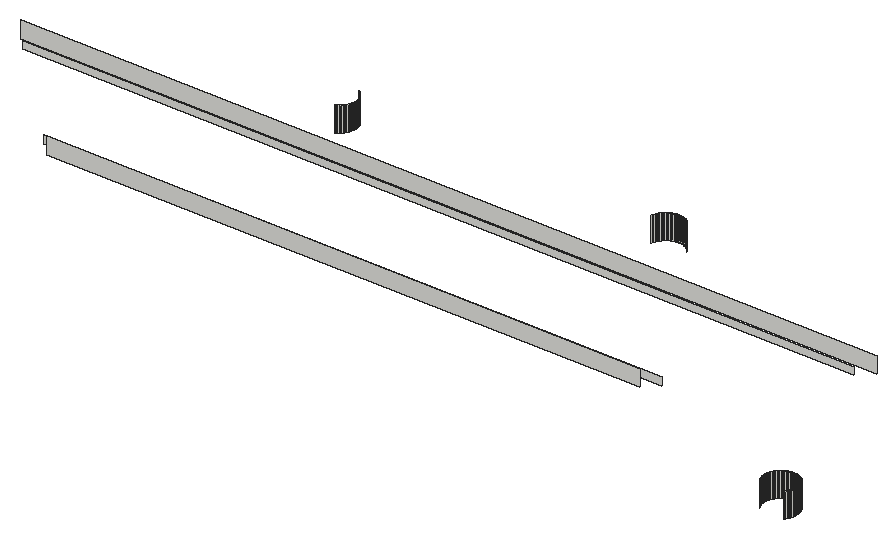
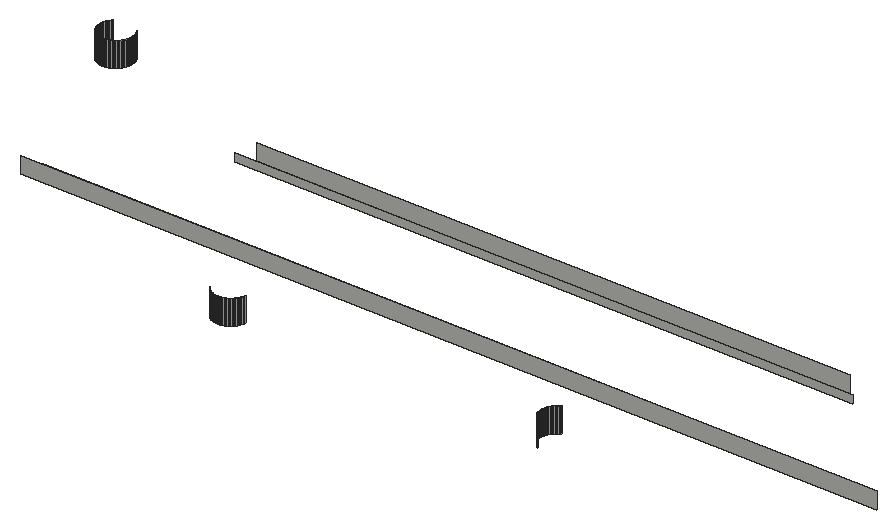
# SketchUp Ruby script. Lengths in millimetres.
U = 1.mm
M = Sketchup.active_model
def pt(a) = Geom::Point3d.new(a.map { |v| v * U })
def face(e, loops, mat)
  f = e.add_face(loops[0].map { |a| pt(a) })
  loops[1..].each { |l| e.add_face(l.map { |a| pt(a) }).erase! }
  f.material = f.back_material = mat if mat
  f
end
# faces: each face lists its corners as indices into pts; further lists are holes
def faces(e, pts, list, mat = nil) = list.each { |f| face(e, (f[0].is_a?(Array) ? f : [f]).map { |l| l.map { |i| pts[i] } }, mat) }
# xy, xz, yz: faces in a plane at the given z, y or x. An outline is a flat list of corners, or four numbers for a rectangle; further outlines are holes
def ring(l) = l.size == 4 ? [[l[0], l[1]], [l[2], l[1]], [l[2], l[3]], [l[0], l[3]]] : l.each_slice(2).to_a
def flat(e, list, mat, &to3) = list.each { |f| face(e, (f[0].is_a?(Array) ? f : [f]).map { |l| ring(l).map { |u, v| to3.(u, v) } }, mat) }
def xy(e, z, list, mat = nil) = flat(e, list, mat) { |x, y| [x, y, z] }
def xz(e, y, list, mat = nil) = flat(e, list, mat) { |x, z| [x, y, z] }
def yz(e, x, list, mat = nil) = flat(e, list, mat) { |y, z| [x, y, z] }
def lines(e, pts, list) = list.each { |a, b| e.add_line(pt(pts[a]), pt(pts[b])) }
# prism: a flat outline (further loops are holes) pulled along v
def prism(e, loops, v, mat = nil)
  f = face(e, loops, mat); d = Geom::Vector3d.new(v.map { |x| x * U })
  f.pushpull(f.normal.samedirection?(d) ? d.length : -d.length)
end
def box(e, o, s, mat = nil) = prism(e, [[o, [o[0] + s[0], o[1], o[2]], [o[0] + s[0], o[1] + s[1], o[2]], [o[0], o[1] + s[1], o[2]]]], [0, 0, s[2]], mat)
def at(x, y, z, deg = 0) = Geom::Transformation.translation(pt([x, y, z])) * Geom::Transformation.rotation(ORIGIN, Z_AXIS, deg.degrees)
def axes(o, x, y, z) = Geom::Transformation.new([*x, 0, *y, 0, *z, 0, *pt(o).to_a, 1])
def part(name) = M.definitions.add(name)
# library, detail: a bought-in or finely detailed component or shape, given as its bounding box
def library(name, o, s) = part(name).tap { |d| box(d.entities, o, s) }
def detail(e, o, s) = box(e.add_group.entities, o, s)
def put(e, d, t, mat = nil) = e.add_instance(d, t).tap { |i| i.material = mat if mat }
def group(e, t, mat = nil) = e.add_group.tap { |g| g.transformation = t; g.material = mat if mat }.entities
root = M.entities
xz(root,2082.8,[[1041.4,2743.2,2870.8,2794]])
xz(root,2120.9,[[1003.3,2743.2,2908.9,2768.6]])
xz(root,2451.1,[[673.1,2743.2,3239.1,2766.6]])
xz(root,2489.2,[[635,2743.2,3277.2,2794]])
p = [[3519.2,1829.2,2718.2],[3519.2,1829.2,2794],[3521.3,1831.6,2794],[3521.3,1831.6,2718.2],[3441.1,1834.1,2718.2],[3441.1,1834.1,2794],
  [3443.1,1831.6,2794],[3443.1,1831.6,2718.2],[3523.3,1834.1,2794],[3523.3,1834.1,2718.2],[3439.3,1836.7,2718.2],[3439.3,1836.7,2794],
  [3525.1,1836.7,2794],[3525.1,1836.7,2718.2],[3437.7,1839.5,2718.2],[3437.7,1839.5,2794],[3526.7,1839.5,2794],[3526.7,1839.5,2718.2],
  [3436.2,1842.3,2718.2],[3436.2,1842.3,2794],[3528.2,1842.3,2794],[3528.2,1842.3,2718.2],[3435,1845.2,2718.2],[3435,1845.2,2794],
  [3529.4,1845.2,2794],[3529.4,1845.2,2718.2],[3433.9,1848.2,2718.2],[3433.9,1848.2,2794],[3530.5,1848.2,2794],[3530.5,1848.2,2718.2],
  [3433,1851.3,2718.2],[3433,1851.3,2794],[3531.4,1851.3,2794],[3531.4,1851.3,2718.2],[3432.3,1854.4,2718.2],[3432.3,1854.4,2794],
  [3532.1,1854.4,2794],[3532.1,1854.4,2718.2],[3431.8,1857.6,2718.2],[3431.8,1857.6,2794],[3532.6,1857.6,2794],[3532.6,1857.6,2718.2],
  [3431.5,1860.7,2718.2],[3431.5,1860.7,2794],[3532.9,1860.7,2794],[3532.9,1860.7,2718.2],[3431.4,1863.9,2718.2],[3431.4,1863.9,2794],
  [3533,1863.9,2794],[3533,1863.9,2718.2],[3431.5,1867.1,2718.2],[3431.5,1867.1,2794],[3532.9,1867.1,2794],[3532.9,1867.1,2718.2],
  [3431.8,1870.3,2718.2],[3431.8,1870.3,2794],[3532.6,1870.3,2794],[3532.6,1870.3,2718.2],[3432.3,1873.5,2718.2],[3432.3,1873.5,2794],
  [3532.1,1873.5,2794],[3532.1,1873.5,2718.2],[3433,1876.6,2718.2],[3433,1876.6,2794],[3531.4,1876.6,2794],[3531.4,1876.6,2718.2],
  [3433.9,1879.6,2718.2],[3433.9,1879.6,2794],[3530.5,1879.6,2794],[3530.5,1879.6,2718.2],[3435,1882.6,2718.2],[3435,1882.6,2794],
  [3529.4,1882.6,2794],[3529.4,1882.6,2718.2],[3436.2,1885.6,2718.2],[3436.2,1885.6,2794],[3528.2,1885.6,2794],[3528.2,1885.6,2718.2],
  [3437.7,1888.4,2718.2],[3437.7,1888.4,2794],[3526.7,1888.4,2794],[3526.7,1888.4,2718.2],[3439.3,1891.2,2718.2],[3439.3,1891.2,2794],
  [3525.1,1891.2,2794],[3525.1,1891.2,2718.2],[3441.1,1893.8,2718.2],[3441.1,1893.8,2794],[3523.3,1893.8,2794],[3523.3,1893.8,2718.2],
  [3443.1,1896.3,2718.2],[3443.1,1896.3,2794],[3521.3,1896.3,2794],[3521.3,1896.3,2718.2],[3445.2,1898.7,2718.2],[3445.2,1898.7,2794],
  [3519.2,1898.7,2794],[3519.2,1898.7,2718.2],[3447.4,1901,2718.2],[3447.4,1901,2794],[3517,1901,2794],[3517,1901,2718.2],
  [3449.8,1903.1,2718.2],[3449.8,1903.1,2794],[3514.6,1903.1,2794],[3514.6,1903.1,2718.2],[3452.3,1905,2718.2],[3452.3,1905,2794],
  [3512.1,1905,2794],[3512.1,1905,2718.2],[3455,1906.8,2718.2],[3455,1906.8,2794],[3509.4,1906.8,2794],[3509.4,1906.8,2718.2],
  [3457.7,1908.4,2718.2],[3457.7,1908.4,2794],[3506.7,1908.4,2794],[3506.7,1908.4,2718.2],[3460.6,1909.9,2718.2],[3460.6,1909.9,2794],
  [3503.8,1909.9,2794],[3503.8,1909.9,2718.2],[3463.5,1911.2,2718.2],[3463.5,1911.2,2794],[3500.9,1911.2,2794],[3500.9,1911.2,2718.2],
  [3466.5,1912.2,2718.2],[3466.5,1912.2,2794],[3497.9,1912.2,2794],[3497.9,1912.2,2718.2],[3469.6,1913.1,2718.2],[3469.6,1913.1,2794],
  [3494.8,1913.1,2794],[3494.8,1913.1,2718.2],[3472.7,1913.8,2718.2],[3472.7,1913.8,2794],[3491.7,1913.8,2794],[3491.7,1913.8,2718.2],
  [3475.8,1914.3,2718.2],[3475.8,1914.3,2794],[3488.6,1914.3,2794],[3488.6,1914.3,2718.2],[3479,1914.6,2718.2],[3479,1914.6,2794],
  [3485.4,1914.6,2794],[3485.4,1914.6,2718.2],[3482.2,1914.7,2718.2],[3482.2,1914.7,2794],[1490,2637.1,2794],[1490,2637.1,2718.2],
  [1487.2,2635.6,2718.2],[1487.2,2635.6,2794],[1492.8,2638.7,2794],[1492.8,2638.7,2718.2],[1495.4,2640.5,2794],[1495.4,2640.5,2718.2],
  [1497.9,2642.5,2794],[1497.9,2642.5,2718.2],[1500.3,2644.6,2794],[1500.3,2644.6,2718.2],[1502.6,2646.8,2794],[1502.6,2646.8,2718.2],
  [1504.7,2649.2,2794],[1504.7,2649.2,2718.2],[1506.6,2651.7,2794],[1506.6,2651.7,2718.2],[1508.4,2654.4,2794],[1508.4,2654.4,2718.2],
  [1510,2657.1,2794],[1510,2657.1,2718.2],[1511.5,2660,2794],[1511.5,2660,2718.2],[1512.8,2662.9,2794],[1512.8,2662.9,2718.2],
  [1513.8,2665.9,2794],[1513.8,2665.9,2718.2],[1514.7,2669,2794],[1514.7,2669,2718.2],[1515.4,2672.1,2794],[1515.4,2672.1,2718.2],
  [1515.9,2675.2,2794],[1515.9,2675.2,2718.2],[1516.2,2678.4,2794],[1516.2,2678.4,2718.2],[1516.3,2681.6,2794],[1516.3,2681.6,2718.2],
  [1516.2,2684.8,2794],[1516.2,2684.8,2718.2],[1515.9,2688,2794],[1515.9,2688,2718.2],[1515.4,2691.1,2794],[1515.4,2691.1,2718.2],
  [2424,2691.1,2718.2],[2424,2691.1,2794],[2423.5,2688,2794],[2423.5,2688,2718.2],[1514.7,2694.2,2794],[1514.7,2694.2,2718.2],
  [2424.7,2694.2,2718.2],[2424.7,2694.2,2794],[1513.8,2697.3,2794],[1513.8,2697.3,2718.2],[2425.6,2697.3,2718.2],[2425.6,2697.3,2794],
  [1512.8,2700.3,2794],[1512.8,2700.3,2718.2],[2426.6,2700.3,2718.2],[2426.6,2700.3,2794],[1511.5,2703.2,2794],[1511.5,2703.2,2718.2],
  [2427.9,2703.2,2718.2],[2427.9,2703.2,2794],[1510,2706.1,2794],[1510,2706.1,2718.2],[2429.4,2706.1,2718.2],[2429.4,2706.1,2794],
  [2431,2708.8,2718.2],[2431,2708.8,2794],[2518.4,2706.1,2718.2],[2518.4,2706.1,2794],[2516.8,2708.8,2794],[2516.8,2708.8,2718.2],
  [2432.8,2711.5,2718.2],[2432.8,2711.5,2794],[2515,2711.5,2794],[2515,2711.5,2718.2],[2434.7,2714,2718.2],[2434.7,2714,2794],
  [2513,2714,2794],[2513,2714,2718.2],[2436.8,2716.4,2718.2],[2436.8,2716.4,2794],[2510.9,2716.4,2794],[2510.9,2716.4,2718.2],
  [2439.1,2718.6,2718.2],[2439.1,2718.6,2794],[2508.6,2718.6,2794],[2508.6,2718.6,2718.2],[1497.9,2720.7,2794],[1497.9,2720.7,2718.2],
  [1500.3,2718.6,2718.2],[1500.3,2718.6,2794],[2441.5,2720.7,2718.2],[2441.5,2720.7,2794],[2506.2,2720.7,2794],[2506.2,2720.7,2718.2],
  [1495.4,2722.7,2794],[1495.4,2722.7,2718.2],[2444,2722.7,2718.2],[2444,2722.7,2794],[2503.7,2722.7,2794],[2503.7,2722.7,2718.2],
  [1492.8,2724.5,2794],[1492.8,2724.5,2718.2],[2446.6,2724.5,2718.2],[2446.6,2724.5,2794],[2501.1,2724.5,2794],[2501.1,2724.5,2718.2],
  [1490,2726.1,2794],[1490,2726.1,2718.2],[2449.4,2726.1,2718.2],[2449.4,2726.1,2794],[2498.3,2726.1,2794],[2498.3,2726.1,2718.2],
  [2452.2,2727.6,2718.2],[2452.2,2727.6,2794],[2495.5,2727.6,2794],[2495.5,2727.6,2718.2],[2455.2,2728.8,2718.2],[2455.2,2728.8,2794],
  [2492.6,2728.8,2794],[2492.6,2728.8,2718.2],[2458.2,2729.9,2718.2],[2458.2,2729.9,2794],[2489.6,2729.9,2794],[2489.6,2729.9,2718.2],
  [2461.2,2730.8,2718.2],[2461.2,2730.8,2794],[2486.5,2730.8,2794],[2486.5,2730.8,2718.2],[2464.3,2731.5,2718.2],[2464.3,2731.5,2794],
  [2483.4,2731.5,2794],[2483.4,2731.5,2718.2],[2467.5,2732,2718.2],[2467.5,2732,2794],[2480.2,2732,2794],[2480.2,2732,2718.2],
  [2470.7,2732.3,2718.2],[2470.7,2732.3,2794],[2477.1,2732.3,2794],[2477.1,2732.3,2718.2],[2473.9,2732.4,2718.2],[2473.9,2732.4,2794]]
faces(root,p,[[0,1,2,3],[4,5,6,7],[3,2,8,9],[10,11,5,4],[9,8,12,13],[14,15,11,10],[13,12,16,17],[18,19,15,14],
  [17,16,20,21],[22,23,19,18],[21,20,24,25],[26,27,23,22],[25,24,28,29],[30,31,27,26],[29,28,32,33],[34,35,31,30],
  [33,32,36,37],[38,39,35,34],[37,36,40,41],[42,43,39,38],[41,40,44,45],[46,47,43,42],[45,44,48,49],[50,51,47,46],
  [49,48,52,53],[54,55,51,50],[53,52,56,57],[58,59,55,54],[57,56,60,61],[62,63,59,58],[61,60,64,65],[66,67,63,62],
  [65,64,68,69],[70,71,67,66],[69,68,72,73],[74,75,71,70],[73,72,76,77],[78,79,75,74],[77,76,80,81],[82,83,79,78],
  [81,80,84,85],[86,87,83,82],[85,84,88,89],[90,91,87,86],[89,88,92,93],[94,95,91,90],[93,92,96,97],[98,99,95,94],
  [97,96,100,101],[102,103,99,98],[101,100,104,105],[106,107,103,102],[105,104,108,109],[110,111,107,106],[109,108,112,113],[114,115,111,110],
  [113,112,116,117],[118,119,115,114],[117,116,120,121],[122,123,119,118],[121,120,124,125],[126,127,123,122],[125,124,128,129],[130,131,127,126],
  [129,128,132,133],[134,135,131,130],[133,132,136,137],[138,139,135,134],[137,136,140,141],[142,143,139,138],[141,140,144,145],[146,147,143,142],
  [145,144,147,146],[148,149,150,151],[152,153,149,148],[154,155,153,152],[156,157,155,154],[158,159,157,156],[160,161,159,158],[162,163,161,160],
  [164,165,163,162],[166,167,165,164],[168,169,167,166],[170,171,169,168],[172,173,171,170],[174,175,173,172],[176,177,175,174],[178,179,177,176],
  [180,181,179,178],[182,183,181,180],[184,185,183,182],[186,187,185,184],[188,189,187,186],[190,191,189,188],[192,193,194,195],[196,197,191,190],
  [198,199,193,192],[200,201,197,196],[202,203,199,198],[204,205,201,200],[206,207,203,202],[208,209,205,204],[210,211,207,206],[212,213,209,208],
  [214,215,211,210],[216,217,215,214],[218,219,220,221],[222,223,217,216],[221,220,224,225],[226,227,223,222],[225,224,228,229],[230,231,227,226],
  [229,228,232,233],[234,235,231,230],[233,232,236,237],[238,239,240,241],[242,243,235,234],[237,236,244,245],[246,247,239,238],[248,249,243,242],
  [245,244,250,251],[252,253,247,246],[254,255,249,248],[251,250,256,257],[258,259,253,252],[260,261,255,254],[257,256,262,263],[264,265,261,260],
  [263,262,266,267],[268,269,265,264],[267,266,270,271],[272,273,269,268],[271,270,274,275],[276,277,273,272],[275,274,278,279],[280,281,277,276],
  [279,278,282,283],[284,285,281,280],[283,282,286,287],[288,289,285,284],[287,286,290,291],[292,293,289,288],[291,290,293,292]])
